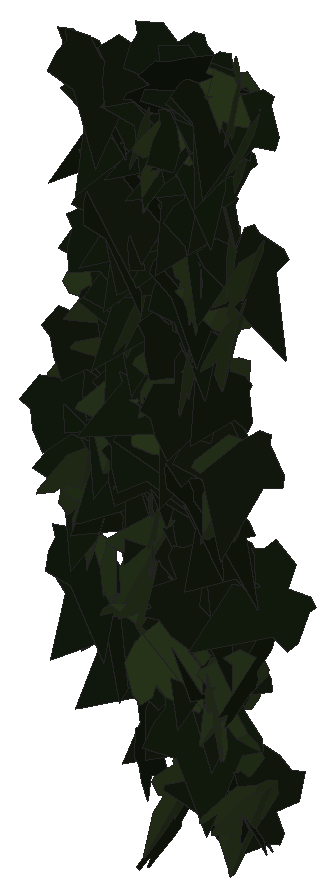
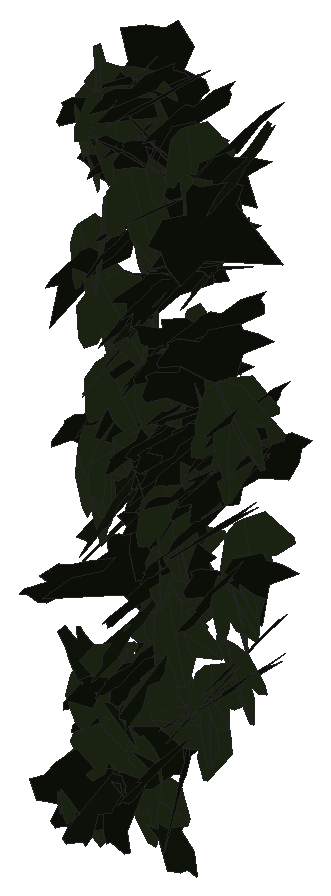
# SketchUp Ruby script. Lengths in inches.
U = 1.inch
M = Sketchup.active_model
def pt(a) = Geom::Point3d.new(a.map { |v| v * U })
def face(e, loops, mat)
  f = e.add_face(loops[0].map { |a| pt(a) })
  loops[1..].each { |l| e.add_face(l.map { |a| pt(a) }).erase! }
  f.material = f.back_material = mat if mat
  f
end
# faces: each face lists its corners as indices into pts; further lists are holes
def faces(e, pts, list, mat = nil) = list.each { |f| face(e, (f[0].is_a?(Array) ? f : [f]).map { |l| l.map { |i| pts[i] } }, mat) }
# xy, xz, yz: faces in a plane at the given z, y or x. An outline is a flat list of corners, or four numbers for a rectangle; further outlines are holes
def ring(l) = l.size == 4 ? [[l[0], l[1]], [l[2], l[1]], [l[2], l[3]], [l[0], l[3]]] : l.each_slice(2).to_a
def flat(e, list, mat, &to3) = list.each { |f| face(e, (f[0].is_a?(Array) ? f : [f]).map { |l| ring(l).map { |u, v| to3.(u, v) } }, mat) }
def xy(e, z, list, mat = nil) = flat(e, list, mat) { |x, y| [x, y, z] }
def xz(e, y, list, mat = nil) = flat(e, list, mat) { |x, z| [x, y, z] }
def yz(e, x, list, mat = nil) = flat(e, list, mat) { |y, z| [x, y, z] }
def lines(e, pts, list) = list.each { |a, b| e.add_line(pt(pts[a]), pt(pts[b])) }
# prism: a flat outline (further loops are holes) pulled along v
def prism(e, loops, v, mat = nil)
  f = face(e, loops, mat); d = Geom::Vector3d.new(v.map { |x| x * U })
  f.pushpull(f.normal.samedirection?(d) ? d.length : -d.length)
end
def box(e, o, s, mat = nil) = prism(e, [[o, [o[0] + s[0], o[1], o[2]], [o[0] + s[0], o[1] + s[1], o[2]], [o[0], o[1] + s[1], o[2]]]], [0, 0, s[2]], mat)
def at(x, y, z, deg = 0) = Geom::Transformation.translation(pt([x, y, z])) * Geom::Transformation.rotation(ORIGIN, Z_AXIS, deg.degrees)
def axes(o, x, y, z) = Geom::Transformation.new([*x, 0, *y, 0, *z, 0, *pt(o).to_a, 1])
def part(name) = M.definitions.add(name)
# library, detail: a bought-in or finely detailed component or shape, given as its bounding box
def library(name, o, s) = part(name).tap { |d| box(d.entities, o, s) }
def detail(e, o, s) = box(e.add_group.entities, o, s)
def put(e, d, t, mat = nil) = e.add_instance(d, t).tap { |i| i.material = mat if mat }
def group(e, t, mat = nil) = e.add_group.tap { |g| g.transformation = t; g.material = mat if mat }.entities
root = M.entities
M.materials.add("efeu1").color = [18, 25, 13]
M.materials.add("efeu2").color = [43, 57, 29]
c1 = part("ivyleaf_10")
p = [[0,0.5,-0.03],[-0.0625,2.02,-0.43],[-0.19,2.01,-0.46],[-0.54,1.05,-0.29],[-0.52,0.625,-0.18],[-0.83,0.76,-0.28],
  [-1.16,0.64,-0.33],[-1.15,0.33,-0.24],[-0.77,-0.39,0.02],[-0.3,-0.51,0.16],[0.04,-0.48,0.23],[-0.02,2.01,-0.4375],
  [-0.06,2.01,-0.43],[0.04,-0.49,0.23],[0.67,-0.49,0.14],[1.38,0.36,-0.2],[1.375,0.51,-0.24],[0.81,0.65,-0.19],
  [0.62,0.59,-0.15],[0.6,1.09,-0.28],[0.5,1.23,-0.31]]
faces(c1.entities,p,[[0,1,2,3,4,5,6,7,8,9,10],[11,12,0,13,14,15,16,17,18,19,20]],"efeu2")
c2 = part("ivyleaf_9")
p = [[1.54,2.16,1.25],[1.36,2.04,1.19],[-0.21,0.99,0.68],[-0.71,1.11,0.82],[-0.85,0.86,0.67],[-0.8,0.17,0.21],
  [-0.9,-0.01,0.1],[-0.67,-0.16,-0.02],[-0.08,-0.08,-0.05],[-0.03,-0.6,-0.4],[0.65,-0.88,-0.66],[0.83,-0.6,-0.49],
  [1.29,-0.42,-0.43],[1.8125,-0.07,-0.26],[1.21,0.44,0.15]]
faces(c2.entities,p,[[0,1,2,3,4,5,6,7,8,9,10,11,12,13,14]],"efeu1")
put(root,c1,axes([25.8125,223.09,228.51],[-0.1191,-0.44393,0.19683],[0.07022,-0.21628,-0.4453],[0.4805,-0.07843,0.11387]))
put(root,c2,axes([25.62,223.09,231.12],[0.18504,-0.45754,0.08009],[0.0285,-0.07486,-0.49354],[0.46362,0.18722,-0.00163]))
put(root,c2,axes([26.375,223.28,228.64],[-0.36452,-0.20418,0.27465],[-0.09442,-0.32569,-0.36744],[0.32895,-0.31974,0.19889]))
put(root,c2,axes([26.83,223.11,227.65],[0.2048,-0.42596,0.16315],[0.07833,-0.14334,-0.47256],[0.44936,0.21912,0.00802]))
put(root,c1,axes([27.03,222.85,230.69],[0.37605,-0.28672,-0.1624],[-0.0875,0.15069,-0.46865],[0.31769,0.3809,0.06316]))
put(root,c2,axes([25.3125,223.1875,232.99],[0.00584,-0.48596,0.1175],[0.03673,-0.11677,-0.48478],[0.49862,0.01429,0.03433]))
put(root,c1,axes([26.33,223.09,226.7],[-0.12534,-0.43167,0.21899],[-0.05252,-0.21275,-0.44942],[0.48118,-0.13566,0.00799]))
put(root,c1,axes([26.58,222.7,225.3125],[0.14945,0.38967,0.27536],[0.10711,0.25379,-0.41728],[-0.46497,0.18371,-0.00761]))
put(root,c1,axes([26.6,223.23,223.21],[0.07192,-0.33225,0.36666],[0.09589,-0.35413,-0.3397],[0.48542,0.11918,0.01278]))
put(root,c1,axes([26.45,223.15,232.4],[0.05454,-0.43625,0.23814],[0.08356,-0.22811,-0.43702],[0.48994,0.08747,0.04803]))
put(root,c1,axes([27.44,223.2,228.11],[-0.03004,-0.40485,0.29188],[0.08953,-0.29203,-0.39585],[0.491,0.02848,0.09004]))
put(root,c2,axes([27.125,223.28,232.96],[-0.0021,-0.44191,0.2339],[0.0267,-0.23367,-0.44123],[0.49928,0.01063,0.02458]))
put(root,c1,axes([27.02,222.78,229.61],[0.22216,-0.3528,-0.27601],[-0.03132,0.2951,-0.40241],[0.44684,0.19609,0.10901]))
put(root,c2,axes([27.5,223.19,228.33],[-0.13704,-0.48019,-0.02527],[0.00627,0.02449,-0.49936],[0.48081,-0.13718,-0.00069]))
put(root,c2,axes([26.9,222.75,229.14],[0.19821,-0.2388,-0.39203],[-0.07524,0.40434,-0.28434],[0.45283,0.17171,0.12435]))
put(root,c2,axes([27.2,223.35,229.19],[-0.06685,-0.37436,0.32463],[-0.00955,-0.32654,-0.37853],[0.49542,-0.05681,0.03651]))
put(root,c2,axes([25.09,222.8,228.56],[0.09658,-0.26931,-0.41005],[0.02308,0.41995,-0.27038],[0.49004,0.0333,0.09355]))
put(root,c2,axes([25.84,223.4,224.73],[-0.25162,-0.30754,0.30348],[-0.03146,-0.33722,-0.36782],[0.43093,-0.2042,0.15035]))
put(root,c2,axes([26.36,222.86,228.15],[0.0168,-0.2971,-0.4018],[0.00877,0.40214,-0.29699],[0.49964,0.00293,0.01872]))
put(root,c1,axes([27.55,223.02,230.1],[0.10992,-0.48559,-0.04606],[-0.00462,0.04618,-0.49784],[0.48775,0.10987,0.00567]))
put(root,c1,axes([26.09,222.99,229.93],[0.15839,-0.46331,-0.10126],[-0.02186,0.09951,-0.48951],[0.47374,0.1595,0.01126]))
put(root,c2,axes([25.87,223.24,231.4],[-0.14295,-0.47856,-0.02337],[0.00772,0.02208,-0.49945],[0.47907,-0.14315,0.00108]))
put(root,c2,axes([26.6,223.32,230.21],[0.06835,-0.40534,0.28465],[0.12168,-0.2648,-0.40629],[0.48013,0.12482,0.06245]))
put(root,c1,axes([26.47,223.27,229.18],[-0.02882,-0.40816,0.28736],[0.02248,-0.28861,-0.40767],[0.49866,-0.01057,0.03499]))
put(root,c2,axes([26.57,222.72,222.48],[-0.1964,0.45904,-0.02667],[-0.0106,0.02448,0.49929],[0.45969,0.19669,0.00012]))
put(root,c2,axes([26.58,222.68,233.35],[0.34464,0.2365,0.2744],[0.21884,0.16589,-0.41784],[-0.28868,0.4081,0.01084]))
put(root,c2,axes([26.24,222.96,228.23],[0.13075,-0.37353,-0.30558],[-0.00686,0.31512,-0.38814],[0.48255,0.10569,0.07728]))
put(root,c2,axes([26.13,223.37,231.04],[-0.24372,-0.41671,0.1302],[-0.04067,-0.12679,-0.48194],[0.43468,-0.24551,0.02791]))
put(root,c2,axes([26.74,223.12,232.62],[-0.45103,0.21519,0.0164],[-0.03841,-0.04266,-0.49669],[-0.21236,-0.44931,0.05501]))
put(root,c1,axes([27.04,223.12,233.26],[0.48934,0.09112,-0.04733],[-0.04499,-0.01689,-0.49769],[-0.09229,0.49134,-0.00833]))
put(root,c1,axes([25.12,223.11,227.33],[-0.07291,-0.49454,-0.01068],[0.00056,0.01071,-0.49988],[0.49466,-0.07291,-0.00101]))
put(root,c2,axes([26.83,223.25,232.51],[0.01447,-0.49498,-0.06917],[0.00823,0.06943,-0.49509],[0.49972,0.01319,0.01016]))
put(root,c2,axes([27.01,223.25,224.27],[-0.20027,-0.42628,-0.16787],[0.08289,0.14646,-0.47083],[0.45058,-0.21641,0.01201]))
put(root,c2,axes([25.62,223.15,231.41],[0.01436,-0.05352,0.49692],[0.43293,-0.24706,-0.03912],[0.24973,0.43139,0.03924]))
put(root,c2,axes([26.51,223.39,224.89],[0.3304,-0.12679,-0.35322],[0.3199,-0.15091,0.3534],[-0.19623,-0.45951,-0.0186]))
put(root,c2,axes([26.69,223.32,230.24],[0.08098,-0.49278,0.02473],[0.00204,-0.02472,-0.49938],[0.49339,0.08098,-0.00199]))
put(root,c2,axes([26.62,223.46,228.38],[-0.09953,-0.45192,0.18937],[-0.02848,-0.18757,-0.46261],[0.48916,-0.10288,0.0116]))
put(root,c2,axes([26.93,223.44,231.12],[-0.01447,-0.46422,0.18518],[0.00636,-0.18542,-0.46431],[0.49975,-0.01108,0.01127]))
put(root,c1,axes([26.52,222.98,228.25],[0.32351,0.36973,-0.09295],[0.06083,0.07029,0.49128],[0.37635,-0.32918,0.0005]))
put(root,c2,axes([25.625,223.53,227.3],[-0.23405,-0.33313,0.29025],[-0.0116,-0.32371,-0.38089],[0.44169,-0.18503,0.1438]))
put(root,c2,axes([27.11,223.53,226.77],[-0.14444,-0.32256,0.35368],[0.01197,-0.37175,-0.33416],[0.47853,-0.08806,0.11511]))
put(root,c1,axes([26.54,223.1,225.75],[0.15535,0.00803,-0.47519],[-0.46602,0.10062,-0.15066],[0.09321,0.48971,0.03875]))
put(root,c1,axes([27.22,223.47,227.86],[-0.0473,-0.14814,0.4752],[0.26948,-0.40896,-0.10067],[0.4185,0.24659,0.11853]))
put(root,c2,axes([25.17,223.53,225.28],[-0.21941,-0.35311,0.27781],[0.00188,-0.30988,-0.39239],[0.44928,-0.17114,0.13731]))
put(root,c2,axes([26.48,223.15,229.63],[0.23481,-0.41477,-0.1511],[-0.04708,0.14664,-0.47569],[0.43891,0.23762,0.02981]))
put(root,c2,axes([26.1875,222.92,224],[0.2115,-0.10988,-0.43954],[-0.3892,0.20426,-0.23834],[0.23194,0.44295,0.00087]))
put(root,c1,axes([26.17,223.05,232.64],[0.18878,-0.42314,-0.18792],[-0.02222,0.19442,-0.46011],[0.46246,0.18207,0.0546]))
put(root,c2,axes([26.7,223.53,231.49],[-0.2278,-0.402,0.19106],[0.04623,-0.23483,-0.43899],[0.44268,-0.18234,0.14416]))
put(root,c2,axes([24.98,223.375,225.84],[0.09272,-0.48589,0.07292],[0.04754,-0.06499,-0.49347],[0.48902,0.09844,0.03415]))
put(root,c2,axes([25.63,223.45,232.54],[-0.30726,-0.38984,0.06012],[-0.02071,-0.06017,-0.49593],[0.39391,-0.30725,0.02083]))
put(root,c2,axes([26.67,222.97,228.61],[0.29268,0.32235,-0.24582],[-0.22134,-0.12693,-0.43],[-0.33962,0.36052,0.0684]))
put(root,c1,axes([25.99,223.35,227.02],[0.25113,-0.27788,0.33124],[0.29005,-0.1758,-0.36738],[0.32064,0.37667,0.0729]))
put(root,c1,axes([25.32,223.19,226.62],[0.30179,-0.39496,-0.0541],[-0.03247,0.04328,-0.49706],[0.39732,0.30354,0.00048]))
put(root,c2,axes([26.0625,223.48,228.54],[-0.21973,-0.43825,0.09825],[-0.02913,-0.09524,-0.48998],[0.44818,-0.22105,0.01632]))
put(root,c1,axes([27.51,223.14,227.61],[0.0478,-0.48967,-0.08908],[-0.00599,0.08892,-0.49199],[0.49767,0.04811,0.00263]))
put(root,c2,axes([27.29,223.44,233.05],[-0.25913,-0.42737,0.01431],[-0.00023,-0.01659,-0.49972],[0.42761,-0.259,0.0084]))
put(root,c2,axes([26.83,222.89,226.32],[0.19203,-0.04133,-0.4598],[0.07142,0.49466,-0.01464],[0.4561,-0.06005,0.19588]))
put(root,c2,axes([26.16,223.45,230.11],[-0.43599,-0.24329,0.0268],[0.00131,-0.05706,-0.49673],[0.24476,-0.43307,0.05039]))
put(root,c2,axes([26.77,223.37,233.3125],[-0.07552,-0.48503,-0.09508],[0.01649,0.09366,-0.49087],[0.49399,-0.07727,0.00185]))
put(root,c2,axes([26.26,223.23,227],[-0.14429,-0.21029,-0.43007],[0.3567,0.25235,-0.24307],[0.31929,-0.37696,0.0772]))
put(root,c1,axes([25.33,223.18,228.95],[-0.23944,-0.43578,-0.05261],[0.02072,0.04864,-0.4972],[0.43845,-0.24028,-0.00523]))
put(root,c2,axes([25.93,223.51,227.61],[0.06762,-0.40994,0.27817],[0.13731,-0.25424,-0.40805],[0.476,0.13157,0.0782]))
put(root,c1,axes([26.2,223.26,225.92],[0.01473,-0.49976,-0.00514],[-0.00203,0.00508,-0.49997],[0.49978,0.01475,-0.00188]))
put(root,c1,axes([27.59,223.32,223.29],[-0.09513,-0.48082,0.09882],[-0.00647,-0.09942,-0.48997],[0.49082,-0.0945,0.01269]))
put(root,c1,axes([27.07,223.37,229.13],[-0.16199,-0.44324,0.16523],[-0.03982,-0.16125,-0.47161],[0.47135,-0.16595,0.01694]))
put(root,c2,axes([26.3,223.46,232.76],[-0.26117,-0.42239,-0.05812],[0.02363,0.05372,-0.49654],[0.42571,-0.26211,-0.0081]))
put(root,c2,axes([26.3,223.26,230.73],[0.03573,-0.43886,-0.2369],[0.04768,0.23942,-0.43635],[0.49644,0.0086,0.05896]))
put(root,c2,axes([26.11,223.61,231.06],[-0.41352,-0.22332,0.17068],[-0.03673,-0.25808,-0.42666],[0.27866,-0.36541,0.19704]))
put(root,c2,axes([25.03,223.16,229.29],[0.22102,-0.36241,-0.26421],[-0.03349,0.28039,-0.41262],[0.44724,0.2001,0.09967]))
put(root,c1,axes([27.11,223.41,230.2],[-0.24485,-0.37559,0.22133],[-0.07191,-0.21557,-0.44537],[0.42998,-0.24993,0.05155]))
put(root,c2,axes([25.88,223.26,233.31],[0.13707,-0.43392,-0.20719],[-0.00738,0.21352,-0.45206],[0.48079,0.12698,0.05213]))
put(root,c1,axes([27.62,223.36,223.18],[0.01595,-0.49056,0.09537],[-0.00889,-0.09569,-0.49068],[0.49967,0.01396,-0.01178]))
put(root,c2,axes([25.41,223.56,228.2],[-0.11703,-0.47528,0.10205],[-0.01665,-0.10099,-0.48941],[0.48583,-0.11795,0.00781]))
put(root,c2,axes([27.01,223.4,227.26],[0.24857,-0.42992,0.05816],[0.03409,-0.04746,-0.49657],[0.4325,0.25083,0.00571]))
put(root,c1,axes([27.55,223.32,230.82],[0.08796,-0.4922,-0.00073],[0.003,0.00127,-0.49999],[0.49219,0.08795,0.00318]))
put(root,c1,axes([26.97,223.21,232.91],[-0.48148,-0.13466,0.00653],[-0.01007,0.0118,-0.49976],[0.13444,-0.48138,-0.01408]))
put(root,c2,axes([26.29,223.51,233.42],[-0.00232,-0.49921,0.02799],[0.12512,-0.02768,-0.4833],[0.48409,0.00476,0.12505]))
put(root,c2,axes([24.93,223.4375,232.89],[0.23062,-0.4367,0.07814],[0.04635,-0.06387,-0.49373],[0.44121,0.23497,0.01103]))
put(root,c1,axes([27.41,223.46,227.76],[0.14363,-0.44786,0.16969],[0.06756,-0.15643,-0.47007],[0.47414,0.15796,0.01558]))
put(root,c2,axes([27.09,223.5,232.31],[-0.45827,-0.10094,0.17262],[-0.16663,-0.04583,-0.46918],[0.11054,-0.48756,0.00837]))
put(root,c1,axes([27.4375,223.21,233.34],[0.25179,-0.39236,-0.1807],[-0.02208,0.19719,-0.45894],[0.43141,0.23909,0.08198]))
put(root,c2,axes([25.84,223.5625,229.65],[-0.29317,-0.40503,0.00014],[-0.01254,0.0089,-0.49976],[0.40484,-0.29304,-0.01538]))
put(root,c1,axes([26.25,223.26,224.96],[-0.39433,0.0245,-0.30644],[0.30521,-0.02835,-0.39502],[-0.03673,-0.49859,0.0074]))
put(root,c2,axes([25.23,223.37,228.35],[0.1052,-0.45439,-0.18018],[0.00967,0.18621,-0.46393],[0.48871,0.09413,0.04796]))
put(root,c2,axes([27.13,223.4,232.34],[-0.41219,0.18273,0.21612],[-0.24928,-0.05362,-0.4301],[-0.13401,-0.46231,0.1353]))
put(root,c2,axes([25.97,223.44,224.27],[0.30818,-0.28065,0.27615],[0.21728,-0.17123,-0.4165],[0.32835,0.37672,0.01642]))
put(root,c2,axes([25.9,223.69,227.15],[-0.09371,-0.43787,0.22247],[-0.02766,-0.22142,-0.44745],[0.49036,-0.09617,0.01727]))
put(root,c1,axes([25.0625,223.56,226.84],[0.02511,-0.43022,0.25353],[0.07929,-0.2472,-0.42732],[0.49303,0.06167,0.05581]))
put(root,c2,axes([26.54,223.64,225.26],[-0.07314,-0.47878,0.12419],[0.00613,-0.1264,-0.48372],[0.49458,-0.06923,0.02436]))
put(root,c1,axes([27.26,223.6,224.82],[-0.06866,-0.38268,0.3144],[0.00201,-0.31762,-0.38616],[0.49526,-0.05176,0.04516]))
put(root,c1,axes([27.26,223.42,223.99],[-0.24259,-0.11511,0.42178],[-0.3835,-0.1756,-0.2685],[0.20995,-0.45378,-0.00309]))
put(root,c1,axes([27.53,223.4,232.72],[0.19653,-0.45912,-0.02425],[-0.00843,0.02277,-0.49941],[0.45968,0.1967,0.00121]))
put(root,c2,axes([25.85,223.58,229.92],[-0.20041,-0.45385,-0.06211],[0.01801,0.05993,-0.49607],[0.45772,-0.20108,-0.00767]))
put(root,c1,axes([25.1,223.42,225.81],[0.45402,-0.20931,-0.00756],[-0.0041,0.00918,-0.4999],[0.20941,0.45399,0.00662]))
put(root,c1,axes([27.02,223.43,224.77],[-0.0749,0.46261,-0.1743],[0.0422,-0.16966,-0.46844],[-0.49255,-0.08488,-0.01363]))
put(root,c2,axes([25.81,223.71,228.54],[-0.13013,-0.45857,0.15092],[-0.00704,-0.15449,-0.47548],[0.48272,-0.12587,0.03375]))
put(root,c2,axes([25.3,223.4375,230.62],[0.0679,-0.45372,-0.19881],[0.03525,0.20459,-0.45486],[0.49411,0.04775,0.05977]))
put(root,c2,axes([25.41,223.71,225.08],[-0.00017,-0.45218,0.21339],[0.03986,-0.21272,-0.45073],[0.49841,0.01686,0.03612]))
put(root,c2,axes([27.1,223.67,222.97],[0.09992,-0.29718,0.38949],[0.21441,-0.33089,-0.30747],[0.4405,0.22847,0.06131]))
put(root,c1,axes([26.28,223.3,227.16],[0.16023,-0.43166,-0.19491],[0.00927,0.20859,-0.45432],[0.47354,0.14198,0.07485]))
put(root,c2,axes([26.02,223.52,227.77],[0.00158,-0.47959,-0.1414],[-0.01875,0.14124,-0.47927],[0.49965,0.00682,-0.01754]))
put(root,c2,axes([25.05,223.64,227.1],[-0.28752,-0.40436,-0.06185],[0.02628,0.05718,-0.49602],[0.40822,-0.28849,-0.01162]))
put(root,c1,axes([27.34,223.1875,231.2],[0.23315,-0.27167,-0.34905],[-0.06904,0.36738,-0.33206],[0.43689,0.20304,0.1338]))
put(root,c1,axes([26.6,223.52,231.98],[-0.16875,-0.45842,0.10666],[-0.04729,-0.09623,-0.48837],[0.46828,-0.17491,-0.01088]))
put(root,c1,axes([25.17,223.41,229.45],[-0.16068,-0.46849,-0.06853],[0.02724,0.0631,-0.49525],[0.4727,-0.16288,0.00525]))
put(root,c2,axes([26.09,223.49,230.87],[0.14847,-0.45257,-0.15211],[-0.01193,0.15573,-0.47498],[0.4773,0.14467,0.03544]))
put(root,c2,axes([27.73,223.79,226.1],[-0.3566,-0.25685,0.23847],[-0.13784,-0.21001,-0.43232],[0.32224,-0.37407,0.07897]))
put(root,c2,axes([27.59,223.39,225.05],[-0.3565,0.34969,-0.02505],[0.01741,-0.01802,-0.49937],[-0.35015,-0.35692,0.00067]))
put(root,c2,axes([25.55,223.41,228.79],[0.03068,-0.37169,-0.33303],[0.06114,0.33394,-0.36708],[0.4953,-0.0182,0.06594]))
put(root,c1,axes([25.76,223.46,232.88],[-0.041,-0.49475,-0.05952],[0.00536,0.05928,-0.49644],[0.49829,-0.04134,0.00044]))
put(root,c1,axes([26.96,223.46,233.04],[-0.27283,-0.41785,-0.0311],[0.04552,0.00734,-0.49787],[0.41653,-0.2745,0.03404]))
put(root,c2,axes([26.17,223.88,223.83],[-0.186,-0.3023,0.35216],[-0.08067,-0.35256,-0.34525],[0.45705,-0.18525,0.08238]))
put(root,c2,axes([27.25,223.3125,222.8],[0.03627,-0.09795,0.48897],[-0.24816,0.4217,0.10288],[-0.43255,-0.25014,-0.01802]))
put(root,c2,axes([27.59,223.72,222.96],[-0.13582,-0.04414,0.47917],[-0.45611,-0.14686,-0.14281],[0.15335,-0.4759,-0.00037]))
put(root,c2,axes([26.87,223.66,224.9375],[-0.16529,-0.45915,-0.10891],[0.02209,0.10775,-0.48775],[0.47137,-0.16606,-0.01534]))
put(root,c1,axes([25.12,223.52,229.53],[0.4503,-0.12075,-0.18068],[-0.17581,0.04193,-0.46619],[0.12774,0.48339,-0.0047]))
put(root,c1,axes([25.44,223.42,225.25],[-0.02127,-0.47688,-0.14878],[-0.00095,0.14895,-0.4773],[0.49955,-0.02002,-0.00725]))
put(root,c2,axes([26.38,223.89,226.35],[-0.1592,-0.37069,0.29538],[-0.04537,-0.29824,-0.39874],[0.4718,-0.15376,0.06132]))
put(root,c2,axes([27.27,223.48,230.84],[0.1222,-0.41547,-0.24991],[-0.04191,0.24771,-0.4323],[0.48302,0.1266,0.02572]))
put(root,c2,axes([25.24,223.92,226.65],[-0.15847,-0.2862,0.37812],[-0.07173,-0.37962,-0.3174],[0.46877,-0.15485,0.07926]))
put(root,c1,axes([25.37,223.55,224.71],[-0.13406,0.00279,-0.48169],[0.46154,-0.14236,-0.12927],[-0.13787,-0.4793,0.0356]))
put(root,c1,axes([26.03,223.57,227.72],[-0.15116,-0.47513,0.03745],[-0.01147,-0.03565,-0.4986],[0.47647,-0.15159,-0.00012]))
put(root,c2,axes([25.51,223.79,232.11],[-0.07219,0.08305,-0.48774],[0.00605,-0.49272,-0.08479],[-0.49472,-0.01814,0.07013]))
put(root,c2,axes([25.36,223.74,230.34],[-0.25617,-0.42401,-0.06775],[0.04156,0.05404,-0.49533],[0.42738,-0.25941,0.00756]))
put(root,c1,axes([26.35,223.57,223.79],[-0.36363,0.25318,-0.23168],[0.16269,-0.17004,-0.44116],[-0.30217,-0.39622,0.04128]))
put(root,c2,axes([26.53,223.74,225.71],[0.17805,-0.44518,0.1418],[0.07051,-0.12441,-0.47911],[0.46187,0.19061,0.01848]))
